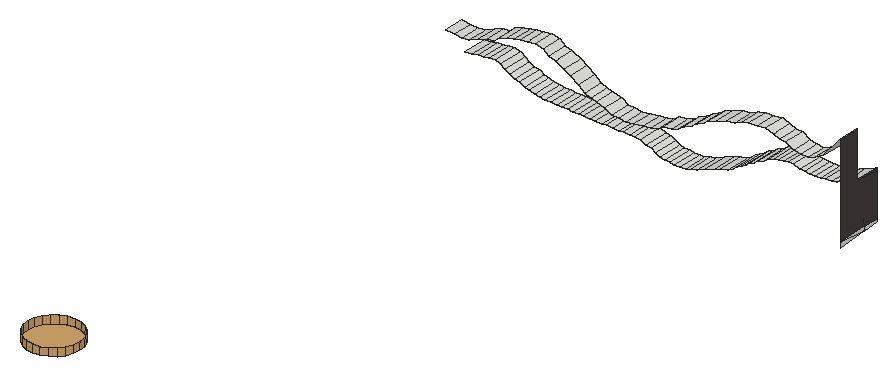
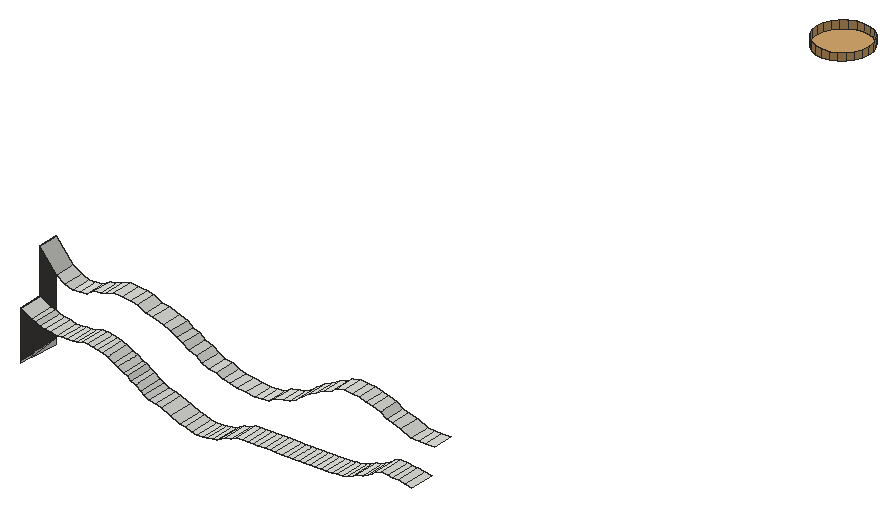
# SketchUp Ruby script. Lengths in inches.
U = 1.inch
M = Sketchup.active_model
def pt(a) = Geom::Point3d.new(a.map { |v| v * U })
def face(e, loops, mat)
  f = e.add_face(loops[0].map { |a| pt(a) })
  loops[1..].each { |l| e.add_face(l.map { |a| pt(a) }).erase! }
  f.material = f.back_material = mat if mat
  f
end
# faces: each face lists its corners as indices into pts; further lists are holes
def faces(e, pts, list, mat = nil) = list.each { |f| face(e, (f[0].is_a?(Array) ? f : [f]).map { |l| l.map { |i| pts[i] } }, mat) }
# xy, xz, yz: faces in a plane at the given z, y or x. An outline is a flat list of corners, or four numbers for a rectangle; further outlines are holes
def ring(l) = l.size == 4 ? [[l[0], l[1]], [l[2], l[1]], [l[2], l[3]], [l[0], l[3]]] : l.each_slice(2).to_a
def flat(e, list, mat, &to3) = list.each { |f| face(e, (f[0].is_a?(Array) ? f : [f]).map { |l| ring(l).map { |u, v| to3.(u, v) } }, mat) }
def xy(e, z, list, mat = nil) = flat(e, list, mat) { |x, y| [x, y, z] }
def xz(e, y, list, mat = nil) = flat(e, list, mat) { |x, z| [x, y, z] }
def yz(e, x, list, mat = nil) = flat(e, list, mat) { |y, z| [x, y, z] }
def lines(e, pts, list) = list.each { |a, b| e.add_line(pt(pts[a]), pt(pts[b])) }
# prism: a flat outline (further loops are holes) pulled along v
def prism(e, loops, v, mat = nil)
  f = face(e, loops, mat); d = Geom::Vector3d.new(v.map { |x| x * U })
  f.pushpull(f.normal.samedirection?(d) ? d.length : -d.length)
end
def box(e, o, s, mat = nil) = prism(e, [[o, [o[0] + s[0], o[1], o[2]], [o[0] + s[0], o[1] + s[1], o[2]], [o[0], o[1] + s[1], o[2]]]], [0, 0, s[2]], mat)
def at(x, y, z, deg = 0) = Geom::Transformation.translation(pt([x, y, z])) * Geom::Transformation.rotation(ORIGIN, Z_AXIS, deg.degrees)
def axes(o, x, y, z) = Geom::Transformation.new([*x, 0, *y, 0, *z, 0, *pt(o).to_a, 1])
def part(name) = M.definitions.add(name)
# library, detail: a bought-in or finely detailed component or shape, given as its bounding box
def library(name, o, s) = part(name).tap { |d| box(d.entities, o, s) }
def detail(e, o, s) = box(e.add_group.entities, o, s)
def put(e, d, t, mat = nil) = e.add_instance(d, t).tap { |i| i.material = mat if mat }
def group(e, t, mat = nil) = e.add_group.tap { |g| g.transformation = t; g.material = mat if mat }.entities
root = M.entities
M.materials.add("[Field Square Tile]").color = [211, 167, 108]
M.materials.add("[Granite Tile]1").color = [68, 65, 63]
xy(root,250.6875,[[1255.793,2328.207,1255.081,2328.3,1254.418,2328.575,1253.848,2329.012,1253.411,2329.582,1253.136,2330.245,1253.043,2330.957,1253.136,2331.668,1253.411,2332.332,1253.848,2332.901,1254.418,2333.338,1255.081,2333.613,1255.793,2333.707,1256.504,2333.613,1257.168,2333.338,1257.737,2332.901,1258.174,2332.332,1258.449,2331.668,1258.543,2330.957,1258.449,2330.245,1258.174,2329.582,1257.737,2329.012,1257.168,2328.575,1256.504,2328.3]],"[Field Square Tile]")
yz(root,1285.595,[[2396.678,240.932,2396.678,241.519,2399.776,241.17],[2399.81,241.167,2399.776,241.17,2399.809,241.173],[2399.776,241.17,2396.678,241.519,2399.769,241.519,2399.809,241.173],[2399.809,241.173,2399.769,241.519,2401.365,241.519,2401.365,241.293]])
yz(root,1285.595,[[2396.678,241.519,2396.678,251.165,2398.803,251.165,2398.803,246.426,2401.365,246.426,2401.365,241.519]],"[Granite Tile]1")
p = [[1266.017,2398.803,241.17],[1266.017,2401.365,241.17],[1266.487,2401.365,241.121],[1266.487,2398.803,241.121],[1267.093,2401.365,241.09],[1267.093,2398.803,241.09],
  [1267.66,2401.365,241.138],[1267.66,2398.803,241.138],[1268.3,2401.365,241.346],[1268.3,2398.803,241.346],[1265.019,2398.803,241.332],[1265.019,2401.365,241.332],
  [1265.487,2401.365,241.243],[1265.487,2398.803,241.243],[1264.6,2398.803,241.566],[1264.6,2401.365,241.566],[1268.891,2401.365,241.456],[1268.891,2398.803,241.456],
  [1269.826,2401.365,241.847],[1269.826,2398.803,241.847],[1264.094,2398.803,241.837],[1264.094,2401.365,241.837],[1263.521,2398.803,241.967],[1263.521,2401.365,241.967],
  [1270.831,2401.365,242.229],[1270.831,2398.803,242.229],[1262.94,2398.803,242.199],[1262.94,2401.365,242.199],[1262.314,2398.803,242.277],[1262.314,2401.365,242.277],
  [1271.392,2401.365,242.424],[1271.392,2398.803,242.424],[1256.467,2398.803,242.35],[1256.467,2401.365,242.35],[1257.049,2401.365,242.342],[1257.049,2398.803,242.342],
  [1257.631,2401.365,242.334],[1257.631,2398.803,242.334],[1258.213,2401.365,242.326],[1258.213,2398.803,242.326],[1258.933,2401.365,242.317],[1258.933,2398.803,242.317],
  [1259.403,2401.365,242.312],[1259.403,2398.803,242.312],[1260.044,2401.365,242.304],[1260.044,2398.803,242.304],[1260.708,2401.365,242.296],[1260.708,2398.803,242.296],
  [1261.16,2401.365,242.291],[1261.16,2398.803,242.291],[1261.798,2401.365,242.283],[1261.798,2398.803,242.283],[1252.985,2398.803,242.466],[1252.985,2401.365,242.466],
  [1253.561,2401.365,242.428],[1253.561,2398.803,242.428],[1254.14,2401.365,242.403],[1254.14,2398.803,242.403],[1254.72,2401.365,242.385],[1254.72,2398.803,242.385],
  [1255.302,2401.365,242.371],[1255.302,2398.803,242.371],[1255.884,2401.365,242.36],[1255.884,2398.803,242.36],[1272.11,2401.365,242.605],[1272.11,2398.803,242.605],
  [1251.857,2398.803,242.599],[1251.857,2401.365,242.599],[1252.417,2401.365,242.518],[1252.417,2398.803,242.518],[1251.304,2398.803,242.75],[1251.304,2401.365,242.75],
  [1272.623,2401.365,242.907],[1272.623,2398.803,242.907],[1250.816,2398.803,242.921],[1250.816,2401.365,242.921],[1250.325,2398.803,243.216],[1250.325,2401.365,243.216],
  [1272.995,2401.365,243.144],[1272.995,2398.803,243.144],[1273.544,2401.365,243.516],[1273.544,2398.803,243.516],[1249.777,2398.803,243.332],[1249.777,2401.365,243.332],
  [1249.232,2398.803,243.589],[1249.232,2401.365,243.589],[1274.018,2401.365,243.711],[1274.018,2398.803,243.711],[1248.751,2398.803,243.88],[1248.751,2401.365,243.88],
  [1274.349,2401.365,244.02],[1274.349,2398.803,244.02],[1248.374,2398.803,244.194],[1248.374,2401.365,244.194],[1244.586,2398.803,243.992],[1244.586,2401.365,243.992],
  [1245.289,2401.365,244.076],[1245.289,2398.803,244.076],[1274.793,2401.365,244.206],[1274.793,2398.803,244.206],[1245.988,2401.365,244.207],[1245.988,2398.803,244.207],
  [1246.573,2401.365,244.266],[1246.573,2398.803,244.266],[1247.777,2398.803,244.387],[1247.777,2401.365,244.387],[1275.382,2401.365,244.569],[1275.382,2398.803,244.569],
  [1247.114,2401.365,244.296],[1247.114,2398.803,244.296],[1275.852,2401.365,244.757],[1275.852,2398.803,244.757],[1276.469,2401.365,245.125],[1276.469,2398.803,245.125],
  [1261.665,2396.678,245.064],[1261.665,2398.803,245.064],[1262.375,2398.803,244.949],[1262.375,2396.678,244.949],[1263.089,2398.803,244.867],[1263.089,2396.678,244.867],
  [1263.995,2398.803,245.007],[1263.995,2396.678,245.007],[1264.939,2398.803,245.121],[1264.939,2396.678,245.121],[1260.952,2396.678,245.459],[1260.952,2398.803,245.459],
  [1265.704,2398.803,245.254],[1265.704,2396.678,245.254],[1276.973,2401.365,245.32],[1276.973,2398.803,245.32],[1280.674,2398.803,245.272],[1280.674,2401.365,245.272],
  [1281.232,2401.365,245.235],[1281.232,2398.803,245.235],[1281.786,2401.365,245.216],[1281.786,2398.803,245.216],[1282.351,2401.365,245.34],[1282.351,2398.803,245.34],
  [1266.456,2398.803,245.41],[1266.456,2396.678,245.41],[1277.455,2401.365,245.411],[1277.455,2398.803,245.411],[1279.021,2398.803,245.552],[1279.021,2401.365,245.552],
  [1279.629,2401.365,245.346],[1279.629,2398.803,245.346],[1280.123,2401.365,245.309],[1280.123,2398.803,245.309],[1282.983,2401.365,245.423],[1282.983,2398.803,245.423],
  [1267.09,2398.803,245.775],[1267.09,2396.678,245.775],[1278.003,2401.365,245.481],[1278.003,2398.803,245.481],[1283.561,2401.365,245.516],[1283.561,2398.803,245.516],
  [1260.077,2396.678,245.671],[1260.077,2398.803,245.671],[1278.485,2401.365,245.59],[1278.485,2398.803,245.59],[1283.941,2401.365,245.763],[1283.941,2398.803,245.763],
  [1259.402,2396.678,245.834],[1259.402,2398.803,245.834],[1258.814,2396.678,246.129],[1258.814,2398.803,246.129],[1267.886,2398.803,245.88],[1267.886,2396.678,245.88],
  [1284.41,2401.365,245.896],[1284.41,2398.803,245.896],[1268.599,2398.803,246.16],[1268.599,2396.678,246.16],[1285.595,2401.365,246.426],[1285.595,2398.803,246.426],
  [1258.183,2396.678,246.633],[1258.183,2398.803,246.633],[1269.196,2398.803,246.573],[1269.196,2396.678,246.573],[1257.369,2396.678,247.185],[1257.369,2398.803,247.185],
  [1269.986,2398.803,246.902],[1269.986,2396.678,246.902],[1245.192,2396.678,246.79],[1245.192,2398.803,246.79],[1245.971,2398.803,246.747],[1245.971,2396.678,246.747],
  [1246.718,2398.803,246.831],[1246.718,2396.678,246.831],[1244.238,2396.678,246.838],[1244.238,2398.803,246.838],[1247.76,2398.803,247.251],[1247.76,2396.678,247.251],
  [1270.588,2398.803,247.347],[1270.588,2396.678,247.347],[1256.657,2396.678,247.553],[1256.657,2398.803,247.553],[1248.634,2398.803,247.546],[1248.634,2396.678,247.546],
  [1271.262,2398.803,247.615],[1271.262,2396.678,247.615],[1249.296,2398.803,247.657],[1249.296,2396.678,247.657],[1255.766,2396.678,248.059],[1255.766,2398.803,248.059],
  [1271.849,2398.803,248.057],[1271.849,2396.678,248.057],[1249.929,2398.803,248.162],[1249.929,2396.678,248.162],[1255.075,2396.678,248.257],[1255.075,2398.803,248.257],
  [1272.614,2398.803,248.322],[1272.614,2396.678,248.322],[1250.723,2398.803,248.408],[1250.723,2396.678,248.408],[1281.411,2396.678,248.295],[1281.411,2398.803,248.295],
  [1282.12,2398.803,248.218],[1282.12,2396.678,248.218],[1282.937,2398.803,248.558],[1282.937,2396.678,248.558],[1254.544,2396.678,248.687],[1254.544,2398.803,248.687],
  [1273.725,2398.803,248.655],[1273.725,2396.678,248.655],[1280.7,2396.678,248.42],[1280.7,2398.803,248.42],[1251.422,2398.803,248.521],[1251.422,2396.678,248.521],
  [1279.903,2396.678,248.895],[1279.903,2398.803,248.895],[1252.116,2398.803,248.723],[1252.116,2396.678,248.723],[1283.872,2398.803,249.022],[1283.872,2396.678,249.022],
  [1252.815,2398.803,248.801],[1252.815,2396.678,248.801],[1253.712,2396.678,248.851],[1253.712,2398.803,248.851],[1274.498,2398.803,248.795],[1274.498,2396.678,248.795],
  [1275.361,2398.803,249.194],[1275.361,2396.678,249.194],[1279.199,2396.678,248.962],[1279.199,2398.803,248.962],[1278.56,2396.678,249.206],[1278.56,2398.803,249.206],
  [1285.595,2398.803,251.165],[1285.595,2396.678,251.165],[1276.034,2398.803,249.323],[1276.034,2396.678,249.323],[1277.815,2396.678,249.478],[1277.815,2398.803,249.478],
  [1276.957,2398.803,249.406],[1276.957,2396.678,249.406],[1255.793,2328.207,251.5],[1255.081,2328.3,251.5],[1255.081,2328.3,250.6875],[1255.793,2328.207,250.6875],
  [1256.504,2328.3,251.5],[1256.504,2328.3,250.6875],[1254.418,2328.575,251.5],[1254.418,2328.575,250.6875],[1257.168,2328.575,251.5],[1257.168,2328.575,250.6875],
  [1253.848,2329.012,251.5],[1253.848,2329.012,250.6875],[1257.737,2329.012,251.5],[1257.737,2329.012,250.6875],[1253.411,2329.582,251.5],[1253.411,2329.582,250.6875],
  [1258.174,2329.582,251.5],[1258.174,2329.582,250.6875],[1253.136,2330.245,251.5],[1253.136,2330.245,250.6875],[1258.449,2330.245,251.5],[1258.449,2330.245,250.6875],
  [1253.043,2330.957,251.5],[1253.043,2330.957,250.6875],[1258.543,2330.957,251.5],[1258.543,2330.957,250.6875],[1253.136,2331.668,251.5],[1253.136,2331.668,250.6875],
  [1258.449,2331.668,251.5],[1258.449,2331.668,250.6875],[1253.411,2332.332,251.5],[1253.411,2332.332,250.6875],[1258.174,2332.332,251.5],[1258.174,2332.332,250.6875],
  [1253.848,2332.901,251.5],[1253.848,2332.901,250.6875],[1257.737,2332.901,251.5],[1257.737,2332.901,250.6875],[1254.418,2333.338,251.5],[1254.418,2333.338,250.6875],
  [1257.168,2333.338,251.5],[1257.168,2333.338,250.6875],[1255.081,2333.613,251.5],[1255.081,2333.613,250.6875],[1256.504,2333.613,251.5],[1256.504,2333.613,250.6875],
  [1255.793,2333.707,251.5],[1255.793,2333.707,250.6875],[1285.595,2400.588,246.171],[1285.595,2399.573,246.265],[1285.595,2401.365,246.273],[1285.595,2399.769,241.519],
  [1285.595,2399.667,242.384]]
faces(root,p,[[0,1,2,3],[3,2,4,5],[5,4,6,7],[7,6,8,9],[10,11,12,13],[13,12,1,0],[14,15,11,10],[9,8,16,17],
  [17,16,18,19],[20,21,15,14],[22,23,21,20],[19,18,24,25],[26,27,23,22],[28,29,27,26],[25,24,30,31],[32,33,34,35],
  [35,34,36,37],[37,36,38,39],[39,38,40,41],[41,40,42,43],[43,42,44,45],[45,44,46,47],[47,46,48,49],[49,48,50,51],
  [51,50,29,28],[52,53,54,55],[55,54,56,57],[57,56,58,59],[59,58,60,61],[61,60,62,63],[63,62,33,32],[31,30,64,65],
  [66,67,68,69],[69,68,53,52],[70,71,67,66],[65,64,72,73],[74,75,71,70],[76,77,75,74],[73,72,78,79],[79,78,80,81],
  [82,83,77,76],[84,85,83,82],[81,80,86,87],[88,89,85,84],[87,86,90,91],[92,93,89,88],[94,95,96,97],[91,90,98,99],
  [97,96,100,101],[101,100,102,103],[104,105,93,92],[99,98,106,107],[103,102,108,109],[109,108,105,104],[107,106,110,111],[111,110,112,113],
  [114,115,116,117],[117,116,118,119],[119,118,120,121],[121,120,122,123],[124,125,115,114],[123,122,126,127],[113,112,128,129],[130,131,132,133],
  [133,132,134,135],[135,134,136,137],[127,126,138,139],[129,128,140,141],[142,143,144,145],[145,144,146,147],[147,146,131,130],[137,136,148,149],
  [139,138,150,151],[141,140,152,153],[149,148,154,155],[156,157,125,124],[153,152,158,159],[155,154,160,161],[159,158,143,142],[162,163,157,156],
  [164,165,163,162],[151,150,166,167],[161,160,168,169],[167,166,170,171],[169,168,172,173],[174,175,165,164],[171,170,176,177],[178,179,175,174],
  [177,176,180,181],[182,183,184,185],[185,184,186,187],[188,189,183,182],[187,186,190,191],[181,180,192,193],[194,195,179,178],[191,190,196,197],
  [193,192,198,199],[197,196,200,201],[202,203,195,194],[199,198,204,205],[201,200,206,207],[208,209,203,202],[205,204,210,211],[207,206,212,213],
  [214,215,216,217],[217,216,218,219],[220,221,209,208],[211,210,222,223],[224,225,215,214],[213,212,226,227],[228,229,225,224],[227,226,230,231],
  [219,218,232,233],[231,230,234,235],[236,237,221,220],[223,222,238,239],[235,234,237,236],[239,238,240,241],[242,243,229,228],[244,245,243,242],
  [233,232,246,247],[241,240,248,249],[250,251,245,244],[249,248,252,253],[253,252,251,250]])
faces(root,p,[[254,255,256,257],[258,254,257,259],[255,260,261,256],[262,258,259,263],[260,264,265,261],[266,262,263,267],[264,268,269,265],[270,266,267,271],
  [268,272,273,269],[274,270,271,275],[272,276,277,273],[278,274,275,279],[276,280,281,277],[282,278,279,283],[280,284,285,281],[286,282,283,287],
  [284,288,289,285],[290,286,287,291],[288,292,293,289],[294,290,291,295],[292,296,297,293],[298,294,295,299],[296,300,301,297],[300,298,299,301]],"[Field Square Tile]")
lines(root,p,[[302,303],[304,302],[305,306]])
